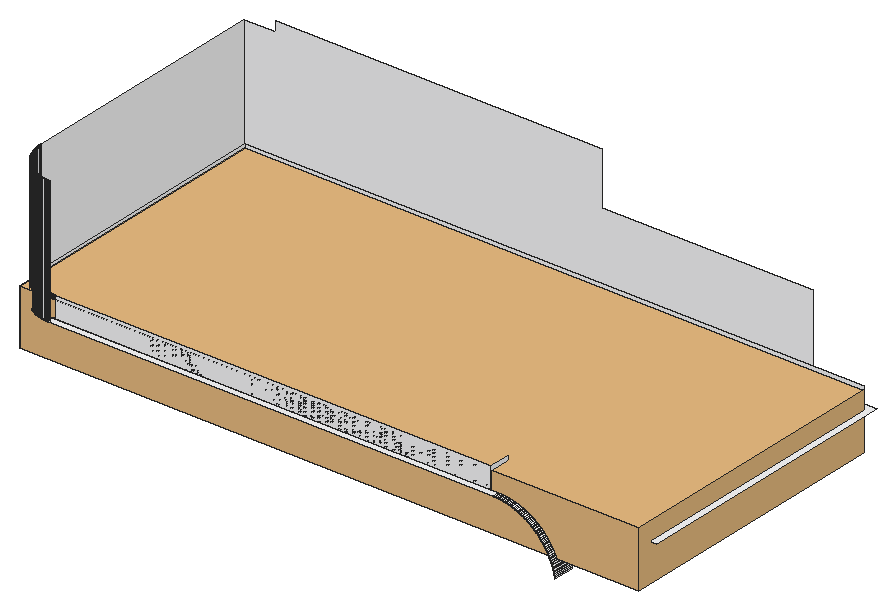
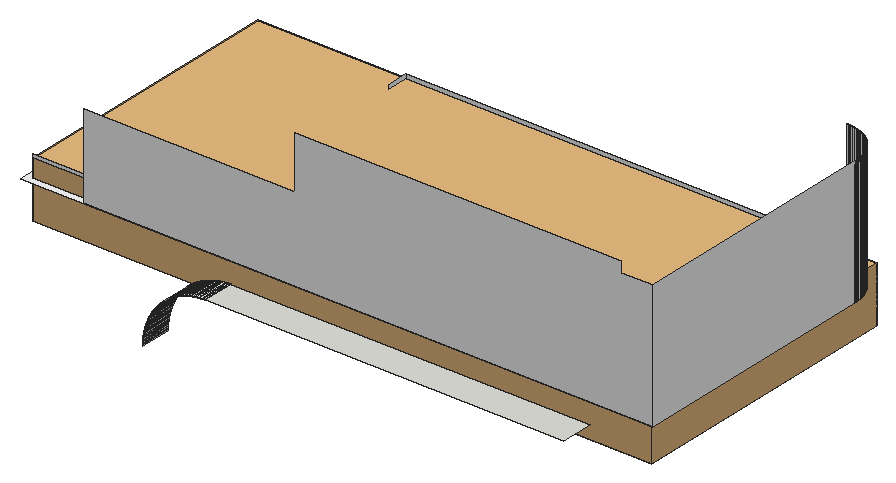
# SketchUp Ruby script. Lengths in inches.
U = 1.inch
M = Sketchup.active_model
def pt(a) = Geom::Point3d.new(a.map { |v| v * U })
def face(e, loops, mat)
  f = e.add_face(loops[0].map { |a| pt(a) })
  loops[1..].each { |l| e.add_face(l.map { |a| pt(a) }).erase! }
  f.material = f.back_material = mat if mat
  f
end
# faces: each face lists its corners as indices into pts; further lists are holes
def faces(e, pts, list, mat = nil) = list.each { |f| face(e, (f[0].is_a?(Array) ? f : [f]).map { |l| l.map { |i| pts[i] } }, mat) }
# xy, xz, yz: faces in a plane at the given z, y or x. An outline is a flat list of corners, or four numbers for a rectangle; further outlines are holes
def ring(l) = l.size == 4 ? [[l[0], l[1]], [l[2], l[1]], [l[2], l[3]], [l[0], l[3]]] : l.each_slice(2).to_a
def flat(e, list, mat, &to3) = list.each { |f| face(e, (f[0].is_a?(Array) ? f : [f]).map { |l| ring(l).map { |u, v| to3.(u, v) } }, mat) }
def xy(e, z, list, mat = nil) = flat(e, list, mat) { |x, y| [x, y, z] }
def xz(e, y, list, mat = nil) = flat(e, list, mat) { |x, z| [x, y, z] }
def yz(e, x, list, mat = nil) = flat(e, list, mat) { |y, z| [x, y, z] }
def lines(e, pts, list) = list.each { |a, b| e.add_line(pt(pts[a]), pt(pts[b])) }
# prism: a flat outline (further loops are holes) pulled along v
def prism(e, loops, v, mat = nil)
  f = face(e, loops, mat); d = Geom::Vector3d.new(v.map { |x| x * U })
  f.pushpull(f.normal.samedirection?(d) ? d.length : -d.length)
end
def box(e, o, s, mat = nil) = prism(e, [[o, [o[0] + s[0], o[1], o[2]], [o[0] + s[0], o[1] + s[1], o[2]], [o[0], o[1] + s[1], o[2]]]], [0, 0, s[2]], mat)
def at(x, y, z, deg = 0) = Geom::Transformation.translation(pt([x, y, z])) * Geom::Transformation.rotation(ORIGIN, Z_AXIS, deg.degrees)
def axes(o, x, y, z) = Geom::Transformation.new([*x, 0, *y, 0, *z, 0, *pt(o).to_a, 1])
def part(name) = M.definitions.add(name)
# library, detail: a bought-in or finely detailed component or shape, given as its bounding box
def library(name, o, s) = part(name).tap { |d| box(d.entities, o, s) }
def detail(e, o, s) = box(e.add_group.entities, o, s)
def put(e, d, t, mat = nil) = e.add_instance(d, t).tap { |i| i.material = mat if mat }
def group(e, t, mat = nil) = e.add_group.tap { |g| g.transformation = t; g.material = mat if mat }.entities
root = M.entities
M.materials.add("[Quartz Light Grey]").color = [251, 251, 252]
c1 = library("Group\#20",[0,0,-16.01],[176,80,16.01])
xy(root,222,[[54,271,156,280],[156,271,156.2,280],[156.2,271,156.4,280]])
xy(root,227.99,[[174.47,187,174.71,193]],"[Quartz Light Grey]")
xy(root,228,[[[47.6875,187,47.53,187.01,47.37,187.02,47.22,187.03,46.9,187.05,46.75,187.07,46.59,187.08,46.43,187.1,46.28,187.125,46.12,187.15,45.97,187.17,45.8125,187.2,45.66,187.23,45.51,187.26,45.35,187.3,45.2,187.33,45.05,187.37,44.89,187.41,44.59,187.49,44.14,187.64,43.99,187.6875,43.85,187.74,43.7,187.8,43.55,187.85,43.41,187.91,43.26,187.97,43.12,188.04,42.98,188.1,42.83,188.17,42.27,188.45,42.14,188.53,42,188.61,41.86,188.6875,41.73,188.77,41.6,188.85,41.46,188.9375,41.33,189.02,41.07,189.2,40.95,189.29,40.82,189.38,40.69,189.48,40.57,189.58,40.45,189.67,40.33,189.77,40.09,189.98,39.97,190.08,39.85,190.1875,39.74,190.3,39.625,190.4,39.51,190.51,39.4,190.625,39.3,190.74,39.1875,190.85,39.08,190.97,38.98,191.09,38.77,191.33,38.67,191.45,38.58,191.57,38.48,191.69,38.38,191.82,38.29,191.95,38.2,192.07,38.02,192.33,37.9375,192.46,37.85,192.6,37.77,192.73,37.6875,192.86,37.61,193,37.53,193.14,37.45,193.27,37.17,193.83,37.1,193.98,37.04,194.12,36.97,194.26,36.91,194.41,36.85,194.55,36.8,194.7,36.74,194.85,36.6875,194.99,36.64,195.14,36.49,195.59,36.41,195.89,36.37,196.05,36.33,196.2,36.3,196.35,36.26,196.51,36.23,196.66,36.2,196.8125,36.17,196.97,36.15,197.12,36.125,197.28,36.1,197.43,36.08,197.59,36.07,197.75,36.05,197.9,36.03,198.22,36.02,198.37,36.01,198.53,36,198.6875,36,271,216,271,216,193,174,193,174,187],[47.74,189,172,189,172,195,214,195,214,269,38,269,38,198.74,38.01,198.61,38.01,198.48,38.03,198.22,38.04,198.08,38.05,197.95,38.09,197.69,38.1,197.57,38.125,197.4375,38.14,197.31,38.17,197.18,38.19,197.05,38.25,196.79,38.28,196.67,38.34,196.41,38.375,196.29,38.41,196.16,38.45,196.03,38.53,195.79,38.57,195.66,38.62,195.54,38.66,195.42,38.71,195.29,38.76,195.17,38.8125,195.05,38.86,194.93,38.92,194.8125,38.97,194.69,39.03,194.58,39.15,194.34,39.21,194.23,39.28,194.11,39.34,194,39.41,193.89,39.47,193.78,39.54,193.66,39.61,193.55,39.69,193.44,39.76,193.34,39.83,193.23,39.91,193.12,39.99,193.02,40.07,192.91,40.23,192.71,40.3125,192.61,40.4,192.51,40.48,192.41,40.66,192.21,40.75,192.12,40.84,192.02,41.02,191.84,41.12,191.75,41.21,191.66,41.41,191.48,41.51,191.4,41.61,191.3125,41.71,191.23,41.91,191.07,42.02,190.99,42.12,190.91,42.23,190.83,42.34,190.76,42.44,190.69,42.55,190.61,42.66,190.54,42.78,190.47,42.89,190.41,43,190.34,43.11,190.28,43.23,190.21,43.34,190.15,43.58,190.03,43.69,189.97,43.8125,189.92,43.93,189.86,44.05,189.8125,44.17,189.76,44.29,189.71,44.42,189.66,44.54,189.62,44.66,189.57,44.79,189.53,45.03,189.45,45.16,189.41,45.29,189.375,45.41,189.34,45.67,189.28,45.79,189.25,46.05,189.19,46.18,189.17,46.31,189.14,46.4375,189.125,46.57,189.1,46.69,189.09,46.95,189.05,47.08,189.04,47.22,189.03,47.48,189.01,47.61,189.01]],[174,187,174.24,193]],"[Quartz Light Grey]")
xz(root,187,[[47.6875,228,47.84,264],[47.84,228,48,264]],"[Quartz Light Grey]")
xz(root,189,[[47.74,228,47.87,234],[47.87,228,48,234],[48,228,172,234]],"[Quartz Light Grey]")
xz(root,189.01,[[47.48,228,47.61,234]],"[Quartz Light Grey]")
xz(root,269,[[38,228,214,234]],"[Quartz Light Grey]")
xz(root,271,[[36,228,36,264,45,264,45,267,138,267,138,252,198,252,198,228]],"[Quartz Light Grey]")
yz(root,36,[[198.6875,228,198.84,264],[198.84,228,199,264],[199,228,271,264]],"[Quartz Light Grey]")
yz(root,38,[[198.74,228,198.87,234],[198.87,228,199,234],[199,228,269,234]],"[Quartz Light Grey]")
yz(root,38.01,[[198.48,228,198.61,234]],"[Quartz Light Grey]")
yz(root,172,[[189,228,195,234]],"[Quartz Light Grey]")
yz(root,174,[[271,204,280,204.2],[271,204.2,280,204.4]])
p = [[174,271,204.4],[173.99,271,204.61],[173.99,280,204.61],[174,280,204.4],[173.98,271,204.81],[173.98,280,204.81],
  [173.97,271,205.01],[173.97,280,205.01],[173.96,271,205.21],[173.96,280,205.21],[173.94,271,205.41],[173.94,280,205.41],
  [173.93,271,205.61],[173.93,280,205.61],[173.91,271,205.81],[173.91,280,205.81],[173.89,271,206.02],[173.89,280,206.02],
  [173.86,271,206.22],[173.86,280,206.22],[173.84,271,206.42],[173.84,280,206.42],[173.81,271,206.62],[173.81,280,206.62],
  [173.78,271,206.82],[173.78,280,206.82],[173.75,271,207.02],[173.75,280,207.02],[173.71,271,207.21],[173.71,280,207.21],
  [173.67,271,207.41],[173.67,280,207.41],[173.63,271,207.61],[173.63,280,207.61],[173.59,271,207.81],[173.59,280,207.81],
  [173.55,271,208.01],[173.55,280,208.01],[173.5,271,208.2],[173.5,280,208.2],[173.45,271,208.4],[173.45,280,208.4],
  [173.4,271,208.59],[173.4,280,208.59],[173.35,271,208.79],[173.35,280,208.79],[173.3,271,208.98],[173.3,280,208.98],
  [173.24,271,209.18],[173.24,280,209.18],[173.18,271,209.37],[173.18,280,209.37],[173.12,271,209.5625],[173.12,280,209.5625],
  [173.06,271,209.75],[173.06,280,209.75],[172.99,271,209.95],[172.99,280,209.95],[172.92,271,210.14],[172.92,280,210.14],
  [172.85,271,210.32],[172.85,280,210.32],[172.78,271,210.51],[172.78,280,210.51],[172.71,271,210.7],[172.71,280,210.7],
  [172.63,271,210.89],[172.63,280,210.89],[172.55,271,211.07],[172.55,280,211.07],[172.47,271,211.26],[172.47,280,211.26],
  [172.39,271,211.44],[172.39,280,211.44],[172.3,271,211.63],[172.3,280,211.63],[172.22,271,211.81],[172.22,280,211.81],
  [172.13,271,211.99],[172.13,280,211.99],[172.04,271,212.17],[172.04,280,212.17],[171.95,271,212.35],[171.95,280,212.35],
  [171.85,271,212.53],[171.85,280,212.53],[171.75,271,212.71],[171.75,280,212.71],[171.66,271,212.88],[171.66,280,212.88],
  [171.55,271,213.06],[171.55,280,213.06],[191.7,187,213.28],[191.7,193,213.28],[191.74,193,213.05],[191.74,187,213.05],
  [171.45,271,213.23],[171.45,280,213.23],[171.35,271,213.4],[171.35,280,213.4],[191.65,187,213.51],[191.65,193,213.51],
  [171.24,271,213.58],[171.24,280,213.58],[191.61,187,213.74],[191.61,193,213.74],[171.13,271,213.75],[171.13,280,213.75],
  [191.56,187,213.97],[191.56,193,213.97],[171.02,271,213.92],[171.02,280,213.92],[170.91,271,214.08],[170.91,280,214.08],
  [191.5,187,214.2],[191.5,193,214.2],[170.8,271,214.25],[170.8,280,214.25],[191.45,187,214.43],[191.45,193,214.43],
  [170.68,271,214.42],[170.68,280,214.42],[191.39,187,214.66],[191.39,193,214.66],[170.5625,271,214.58],[170.5625,280,214.58],
  [170.44,271,214.74],[170.44,280,214.74],[191.32,187,214.89],[191.32,193,214.89],[170.32,271,214.9],[170.32,280,214.9],
  [191.26,187,215.11],[191.26,193,215.11],[170.2,271,215.0625],[170.2,280,215.0625],[191.19,187,215.34],[191.19,193,215.34],
  [170.07,271,215.22],[170.07,280,215.22],[169.95,271,215.38],[169.95,280,215.38],[191.12,187,215.5625],[191.12,193,215.5625],
  [169.82,271,215.54],[169.82,280,215.54],[169.6875,271,215.69],[169.6875,280,215.69],[191.04,187,215.79],[191.04,193,215.79],
  [169.56,271,215.84],[169.56,280,215.84],[190.97,187,216.01],[190.97,193,216.01],[169.42,271,215.99],[169.42,280,215.99],
  [190.89,187,216.23],[190.89,193,216.23],[169.29,271,216.14],[169.29,280,216.14],[169.15,271,216.29],[169.15,280,216.29],
  [190.8,187,216.45],[190.8,193,216.45],[169.01,271,216.4375],[169.01,280,216.4375],[168.87,271,216.58],[168.87,280,216.58],
  [190.72,187,216.67],[190.72,193,216.67],[168.73,271,216.73],[168.73,280,216.73],[190.63,187,216.89],[190.63,193,216.89],
  [168.58,271,216.87],[168.58,280,216.87],[190.54,187,217.11],[190.54,193,217.11],[168.4375,271,217.01],[168.4375,280,217.01],
  [168.29,271,217.15],[168.29,280,217.15],[190.44,187,217.32],[190.44,193,217.32],[168.14,271,217.29],[168.14,280,217.29],
  [190.35,187,217.54],[190.35,193,217.54],[167.99,271,217.42],[167.99,280,217.42],[167.84,271,217.56],[167.84,280,217.56],
  [190.25,187,217.75],[190.25,193,217.75],[167.69,271,217.6875],[167.69,280,217.6875],[190.14,187,217.96],[190.14,193,217.96],
  [167.54,271,217.82],[167.54,280,217.82],[167.38,271,217.95],[167.38,280,217.95],[167.22,271,218.07],[167.22,280,218.07],
  [190.04,187,218.17],[190.04,193,218.17],[167.0625,271,218.2],[167.0625,280,218.2],[189.93,187,218.38],[189.93,193,218.38],
  [166.9,271,218.32],[166.9,280,218.32],[166.74,271,218.44],[166.74,280,218.44],[189.82,187,218.59],[189.82,193,218.59],
  [166.58,271,218.5625],[166.58,280,218.5625],[189.7,187,218.8],[189.7,193,218.8],[166.42,271,218.68],[166.42,280,218.68],
  [166.25,271,218.8],[166.25,280,218.8],[189.59,187,219],[189.59,193,219],[166.08,271,218.91],[166.08,280,218.91],
  [165.92,271,219.02],[165.92,280,219.02],[189.47,187,219.2],[189.47,193,219.2],[165.75,271,219.13],[165.75,280,219.13],
  [165.58,271,219.24],[165.58,280,219.24],[189.35,187,219.4],[189.35,193,219.4],[165.4,271,219.35],[165.4,280,219.35],
  [165.23,271,219.45],[165.23,280,219.45],[189.22,187,219.61],[189.22,193,219.61],[165.06,271,219.55],[165.06,280,219.55],
  [189.1,187,219.8],[189.1,193,219.8],[164.88,271,219.66],[164.88,280,219.66],[164.71,271,219.75],[164.71,280,219.75],
  [188.97,187,220],[188.97,193,220],[164.53,271,219.85],[164.53,280,219.85],[164.35,271,219.95],[164.17,271,220.04],
  [164.17,280,220.04],[164.35,280,219.95],[188.83,187,220.2],[188.83,193,220.2],[163.99,271,220.13],[163.99,280,220.13],
  [163.81,271,220.22],[163.81,280,220.22],[188.7,187,220.39],[188.7,193,220.39],[163.63,271,220.3],[163.63,280,220.3],
  [163.44,271,220.39],[163.44,280,220.39],[188.5625,187,220.58],[188.5625,193,220.58],[163.26,271,220.47],[163.26,280,220.47],
  [163.07,271,220.55],[163.07,280,220.55],[188.42,187,220.77],[188.42,193,220.77],[162.89,271,220.63],[162.7,271,220.71],
  [162.7,280,220.71],[162.89,280,220.63],[162.51,271,220.78],[162.51,280,220.78],[188.28,187,220.96],[188.28,193,220.96],
  [162.32,271,220.85],[162.32,280,220.85],[162.14,271,220.92],[161.95,271,220.99],[161.95,280,220.99],[162.14,280,220.92],
  [188.14,187,221.14],[188.14,193,221.14],[161.75,271,221.06],[161.75,280,221.06],[187.99,187,221.33],[187.99,193,221.33],
  [161.5625,271,221.12],[161.37,271,221.18],[161.37,280,221.18],[161.5625,280,221.12],[161.18,271,221.24],[160.98,271,221.3],
  [160.98,280,221.3],[161.18,280,221.24],[187.84,187,221.51],[187.84,193,221.51],[160.79,271,221.35],[160.79,280,221.35],
  [160.59,271,221.4],[160.4,271,221.45],[160.4,280,221.45],[160.59,280,221.4],[187.6875,187,221.69],[187.6875,193,221.69],
  [160.01,271,221.55],[159.81,271,221.59],[159.81,280,221.59],[160.01,280,221.55],[160.2,271,221.5],[160.2,280,221.5],
  [159.61,271,221.63],[159.41,271,221.67],[159.41,280,221.67],[159.61,280,221.63],[187.53,187,221.87],[187.53,193,221.87],
  [159.02,271,221.75],[158.82,271,221.78],[158.82,280,221.78],[159.02,280,221.75],[159.21,271,221.71],[159.21,280,221.71],
  [158.42,271,221.84],[158.22,271,221.86],[158.22,280,221.86],[158.42,280,221.84],[158.62,271,221.81],[158.62,280,221.81],
  [187.375,187,222.04],[187.375,193,222.04],[157.41,271,221.94],[157.21,271,221.96],[157.21,280,221.96],[157.41,280,221.94],
  [157.61,271,221.93],[157.61,280,221.93],[157.81,271,221.91],[157.81,280,221.91],[158.02,271,221.89],[158.02,280,221.89],
  [187.22,187,222.22],[187.22,193,222.22],[156.61,271,221.99],[156.4,271,222],[156.4,280,222],[156.61,280,221.99],
  [156.81,271,221.98],[156.81,280,221.98],[157.01,271,221.97],[157.01,280,221.97],[187.06,187,222.39],[187.06,193,222.39],
  [186.89,187,222.56],[186.89,193,222.56],[186.73,187,222.73],[186.73,193,222.73],[186.56,187,222.89],[186.56,193,222.89],
  [186.39,187,223.06],[186.39,193,223.06],[186.22,187,223.22],[186.22,193,223.22],[186.04,187,223.375],[186.04,193,223.375],
  [185.87,187,223.53],[185.87,193,223.53],[185.69,187,223.6875],[185.69,193,223.6875],[185.51,187,223.84],[185.51,193,223.84],
  [185.33,187,223.99],[185.33,193,223.99],[185.14,187,224.14],[185.14,193,224.14],[184.96,187,224.28],[184.96,193,224.28],
  [184.77,187,224.42],[184.77,193,224.42],[184.58,187,224.5625],[184.58,193,224.5625],[184.39,187,224.7],[184.39,193,224.7],
  [184.2,187,224.83],[184.2,193,224.83],[184,187,224.97],[184,193,224.97],[183.8,187,225.1],[183.8,193,225.1],
  [183.61,187,225.22],[183.61,193,225.22],[183.4,187,225.35],[183.4,193,225.35],[183.2,187,225.47],[183.2,193,225.47],
  [183,187,225.59],[183,193,225.59],[182.8,187,225.7],[182.8,193,225.7],[182.59,187,225.82],[182.59,193,225.82],
  [182.38,187,225.93],[182.38,193,225.93],[182.17,187,226.04],[182.17,193,226.04],[181.96,187,226.14],[181.96,193,226.14],
  [181.75,187,226.25],[181.75,193,226.25],[181.54,187,226.35],[181.54,193,226.35],[181.32,187,226.44],[181.32,193,226.44],
  [181.11,187,226.54],[181.11,193,226.54],[180.89,187,226.63],[180.89,193,226.63],[180.67,187,226.72],[180.67,193,226.72],
  [180.45,187,226.8],[180.45,193,226.8],[180.23,187,226.89],[180.23,193,226.89],[180.01,187,226.97],[180.01,193,226.97],
  [179.5625,187,227.12],[179.5625,193,227.12],[179.79,193,227.04],[179.79,187,227.04],[179.34,187,227.19],[179.34,193,227.19],
  [179.11,187,227.26],[179.11,193,227.26],[178.66,187,227.39],[178.66,193,227.39],[178.89,193,227.32],[178.89,187,227.32],
  [178.2,187,227.5],[178.2,193,227.5],[178.43,193,227.45],[178.43,187,227.45],[177.97,187,227.56],[177.97,193,227.56],
  [177.51,187,227.65],[177.51,193,227.65],[177.74,193,227.61],[177.74,187,227.61],[176.82,187,227.78],[176.82,193,227.78],
  [177.05,193,227.74],[177.05,187,227.74],[177.28,193,227.7],[177.28,187,227.7],[176.12,187,227.875],[176.12,193,227.875],
  [176.35,193,227.85],[176.35,187,227.85],[176.58,193,227.8125],[176.58,187,227.8125],[175.18,187,227.96],[175.18,193,227.96],
  [175.41,193,227.94],[175.41,187,227.94],[175.65,193,227.92],[175.65,187,227.92],[175.88,193,227.9],[175.88,187,227.9],
  [47.06,187.04,264],[46.9,187.05,264],[46.9,187.05,228],[47.06,187.04,228],[47.22,187.03,264],[47.22,187.03,228],
  [47.37,187.02,264],[47.37,187.02,228],[47.53,187.01,264],[47.53,187.01,228],[47.6875,187,264],[47.6875,187,228],
  [174.24,187,228],[174.24,193,228],[174.47,193,227.99],[174.47,187,227.99],[174.71,187,227.99],[174.71,193,227.99],
  [174.94,193,227.98],[174.94,187,227.98],[46.12,187.15,264],[45.97,187.17,264],[45.97,187.17,228],[46.12,187.15,228],
  [46.28,187.125,264],[46.28,187.125,228],[46.43,187.1,264],[46.43,187.1,228],[46.59,187.08,264],[46.59,187.08,228],
  [46.75,187.07,264],[46.75,187.07,228],[45.66,187.23,264],[45.51,187.26,264],[45.51,187.26,228],[45.66,187.23,228],
  [45.8125,187.2,264],[45.8125,187.2,228],[45.2,187.33,264],[45.05,187.37,264],[45.05,187.37,228],[45.2,187.33,228],
  [45.35,187.3,264],[45.35,187.3,228],[44.89,187.41,264],[44.74,187.45,264],[44.74,187.45,228],[44.89,187.41,228],
  [44.44,187.54,264],[44.29,187.59,264],[44.29,187.59,228],[44.44,187.54,228],[44.59,187.49,264],[44.59,187.49,228],
  [44.14,187.64,264],[43.99,187.6875,264],[43.99,187.6875,228],[44.14,187.64,228],[43.85,187.74,264],[43.7,187.8,264],
  [43.7,187.8,228],[43.85,187.74,228],[43.55,187.85,264],[43.55,187.85,228],[43.41,187.91,264],[43.26,187.97,264],
  [43.26,187.97,228],[43.41,187.91,228],[43.12,188.04,264],[42.98,188.1,264],[42.98,188.1,228],[43.12,188.04,228],
  [42.83,188.17,264],[42.83,188.17,228],[42.69,188.24,264],[42.55,188.31,264],[42.55,188.31,228],[42.69,188.24,228],
  [42.41,188.38,264],[42.41,188.38,228],[42.27,188.45,264],[42.27,188.45,228],[42.14,188.53,264],[42,188.61,264],
  [42,188.61,228],[42.14,188.53,228],[41.86,188.6875,264],[41.86,188.6875,228],[41.73,188.77,264],[41.73,188.77,228],
  [41.6,188.85,264],[41.6,188.85,228],[41.46,188.9375,264],[41.33,189.02,264],[41.33,189.02,228],[41.46,188.9375,228],
  [41.2,189.11,264],[41.2,189.11,228],[47.08,189.04,228],[46.95,189.05,228],[46.95,189.05,234],[47.08,189.04,234],
  [47.22,189.03,228],[47.22,189.03,234],[47.35,189.02,228],[47.35,189.02,234],[47.48,189.01,228],[47.48,189.01,234],
  [47.74,189,228],[47.61,189.01,228],[47.61,189.01,234],[47.74,189,234],[41.07,189.2,264],[41.07,189.2,228],
  [46.31,189.14,228],[46.18,189.17,228],[46.18,189.17,234],[46.31,189.14,234],[46.4375,189.125,228],[46.4375,189.125,234],
  [46.57,189.1,228],[46.57,189.1,234],[46.69,189.09,228],[46.69,189.09,234],[46.82,189.07,228],[46.82,189.07,234],
  [40.95,189.29,264],[40.95,189.29,228],[45.79,189.25,228],[45.67,189.28,228],[45.67,189.28,234],[45.79,189.25,234],
  [45.92,189.22,228],[45.92,189.22,234],[46.05,189.19,228],[46.05,189.19,234],[40.82,189.38,264],[40.82,189.38,228],
  [45.41,189.34,228],[45.29,189.375,228],[45.29,189.375,234],[45.41,189.34,234],[45.54,189.31,228],[45.54,189.31,234],
  [40.69,189.48,264],[40.69,189.48,228],[45.03,189.45,228],[44.91,189.49,228],[44.91,189.49,234],[45.03,189.45,234],
  [45.16,189.41,228],[45.16,189.41,234],[40.57,189.58,264],[40.57,189.58,228],[44.79,189.53,228],[44.66,189.57,228],
  [44.66,189.57,234],[44.79,189.53,234],[40.45,189.67,264],[40.45,189.67,228],[44.54,189.62,228],[44.42,189.66,228],
  [44.42,189.66,234],[44.54,189.62,234],[40.33,189.77,264],[40.33,189.77,228],[44.29,189.71,228],[44.17,189.76,228],
  [44.17,189.76,234],[44.29,189.71,234],[40.21,189.875,264],[40.21,189.875,228],[44.05,189.8125,228],[43.93,189.86,228],
  [43.93,189.86,234],[44.05,189.8125,234],[40.09,189.98,264],[40.09,189.98,228],[43.8125,189.92,228],[43.69,189.97,228],
  [43.69,189.97,234],[43.8125,189.92,234],[39.97,190.08,264],[39.97,190.08,228],[43.58,190.03,228],[43.46,190.09,228],
  [43.46,190.09,234],[43.58,190.03,234],[39.85,190.1875,264],[39.85,190.1875,228],[43.34,190.15,228],[43.34,190.15,234],
  [39.74,190.3,264],[39.74,190.3,228],[43.23,190.21,228],[43.11,190.28,228],[43.11,190.28,234],[43.23,190.21,234],
  [39.625,190.4,264],[39.625,190.4,228],[43,190.34,228],[42.89,190.41,228],[42.89,190.41,234],[43,190.34,234],
  [39.51,190.51,264],[39.51,190.51,228],[42.78,190.47,228],[42.78,190.47,234],[39.4,190.625,264],[39.4,190.625,228],
  [42.66,190.54,228],[42.55,190.61,228],[42.55,190.61,234],[42.66,190.54,234],[39.3,190.74,264],[39.3,190.74,228],
  [42.44,190.69,228],[42.44,190.69,234],[39.1875,190.85,264],[39.1875,190.85,228],[42.34,190.76,228],[42.34,190.76,234],
  [42.23,190.83,228],[42.12,190.91,228],[42.12,190.91,234],[42.23,190.83,234],[39.08,190.97,264],[39.08,190.97,228],
  [42.02,190.99,228],[42.02,190.99,234],[38.98,191.09,264],[38.98,191.09,228],[41.91,191.07,228],[41.91,191.07,234],
  [38.875,191.21,264],[38.875,191.21,228],[41.81,191.15,228],[41.71,191.23,228],[41.71,191.23,234],[41.81,191.15,234],
  [38.77,191.33,264],[38.77,191.33,228],[41.61,191.3125,228],[41.61,191.3125,234],[38.67,191.45,264],[38.67,191.45,228],
  [41.51,191.4,228],[41.51,191.4,234],[38.58,191.57,264],[38.58,191.57,228],[41.41,191.48,228],[41.41,191.48,234],
  [41.31,191.57,228],[41.31,191.57,234],[38.48,191.69,264],[38.48,191.69,228],[41.21,191.66,228],[41.21,191.66,234],
  [38.38,191.82,264],[38.38,191.82,228],[41.12,191.75,228],[41.02,191.84,228],[41.02,191.84,234],[41.12,191.75,234],
  [38.29,191.95,264],[38.29,191.95,228],[40.93,191.93,228],[40.93,191.93,234],[38.2,192.07,264],[38.2,192.07,228],
  [40.84,192.02,228],[40.84,192.02,234],[40.75,192.12,228],[40.75,192.12,234],[38.11,192.2,264],[38.11,192.2,228],
  [40.66,192.21,228],[40.66,192.21,234],[38.02,192.33,264],[38.02,192.33,228],[40.57,192.31,228],[40.57,192.31,234],
  [37.9375,192.46,264],[37.9375,192.46,228],[40.48,192.41,228],[40.48,192.41,234],[40.4,192.51,228],[40.4,192.51,234],
  [37.85,192.6,264],[37.85,192.6,228],[40.3125,192.61,228],[40.3125,192.61,234],[37.77,192.73,264],[37.77,192.73,228],
  [40.23,192.71,228],[40.23,192.71,234],[37.6875,192.86,264],[37.6875,192.86,228],[40.15,192.81,228],[40.15,192.81,234],
  [40.07,192.91,228],[40.07,192.91,234],[37.61,193,264],[37.61,193,228],[39.99,193.02,228],[39.99,193.02,234],
  [37.53,193.14,264],[37.53,193.14,228],[39.91,193.12,228],[39.91,193.12,234],[37.45,193.27,264],[37.45,193.27,228],
  [39.83,193.23,228],[39.83,193.23,234],[39.76,193.34,228],[39.76,193.34,234],[37.38,193.41,264],[37.38,193.41,228],
  [39.69,193.44,228],[39.69,193.44,234],[37.31,193.55,264],[37.31,193.55,228],[39.61,193.55,228],[39.61,193.55,234],
  [37.24,193.69,264],[37.24,193.69,228],[39.54,193.66,228],[39.54,193.66,234],[37.17,193.83,264],[37.17,193.83,228],
  [39.47,193.78,228],[39.47,193.78,234],[37.1,193.98,264],[37.1,193.98,228],[39.41,193.89,228],[39.41,193.89,234],
  [39.34,194,228],[39.34,194,234],[37.04,194.12,264],[37.04,194.12,228],[39.28,194.11,228],[39.28,194.11,234],
  [36.97,194.26,264],[36.97,194.26,228],[39.21,194.23,228],[39.21,194.23,234],[39.15,194.34,228],[39.15,194.34,234],
  [36.91,194.41,264],[36.91,194.41,228],[39.09,194.46,228],[39.09,194.46,234],[36.85,194.55,264],[36.85,194.55,228],
  [39.03,194.58,228],[39.03,194.58,234],[36.8,194.7,264],[36.8,194.7,228],[38.97,194.69,228],[38.97,194.69,234],
  [36.74,194.85,264],[36.74,194.85,228],[38.92,194.8125,228],[38.92,194.8125,234],[36.6875,194.99,264],[36.6875,194.99,228],
  [38.86,194.93,228],[38.86,194.93,234],[38.8125,195.05,228],[38.8125,195.05,234],[36.64,195.14,264],[36.64,195.14,228],
  [36.59,195.29,264],[36.59,195.29,228],[38.76,195.17,228],[38.76,195.17,234],[38.71,195.29,228],[38.71,195.29,234],
  [36.54,195.44,264],[36.54,195.44,228],[38.66,195.42,228],[38.66,195.42,234],[36.49,195.59,264],[36.49,195.59,228],
  [38.62,195.54,228],[38.62,195.54,234],[38.57,195.66,228],[38.57,195.66,234],[36.45,195.74,264],[36.45,195.74,228],
  [36.41,195.89,264],[36.41,195.89,228],[38.53,195.79,228],[38.53,195.79,234],[38.49,195.91,228],[38.49,195.91,234],
  [36.37,196.05,264],[36.37,196.05,228],[38.45,196.03,228],[38.45,196.03,234],[36.33,196.2,264],[36.33,196.2,228],
  [38.41,196.16,228],[38.41,196.16,234],[36.3,196.35,264],[36.3,196.35,228],[38.375,196.29,228],[38.375,196.29,234],
  [38.34,196.41,228],[38.34,196.41,234],[36.26,196.51,264],[36.26,196.51,228],[38.31,196.54,228],[38.31,196.54,234],
  [36.23,196.66,264],[36.23,196.66,228],[38.28,196.67,228],[38.28,196.67,234],[36.2,196.8125,264],[36.2,196.8125,228],
  [38.25,196.79,228],[38.25,196.79,234],[36.17,196.97,264],[36.17,196.97,228],[38.22,196.92,228],[38.22,196.92,234],
  [38.19,197.05,228],[38.19,197.05,234],[36.15,197.12,264],[36.15,197.12,228],[38.17,197.18,228],[38.17,197.18,234],
  [36.125,197.28,264],[36.125,197.28,228],[38.14,197.31,228],[38.14,197.31,234],[36.1,197.43,264],[36.1,197.43,228],
  [38.125,197.4375,228],[38.125,197.4375,234],[36.08,197.59,264],[36.08,197.59,228],[38.1,197.57,228],[38.1,197.57,234],
  [36.07,197.75,264],[36.07,197.75,228],[38.09,197.69,228],[38.09,197.69,234],[36.05,197.9,264],[36.05,197.9,228],
  [38.07,197.82,228],[38.07,197.82,234],[38.05,197.95,228],[38.05,197.95,234],[36.04,198.06,264],[36.04,198.06,228],
  [38.04,198.08,228],[38.04,198.08,234],[36.03,198.22,264],[36.03,198.22,228],[38.03,198.22,228],[38.03,198.22,234],
  [36.02,198.37,264],[36.02,198.37,228],[38.02,198.35,228],[38.02,198.35,234],[38.01,198.48,228],[38.01,198.48,234],
  [36.01,198.53,264],[36.01,198.53,228],[36,198.6875,264],[36,198.6875,228],[38.01,198.61,228],[38,198.74,228],
  [38,198.74,234],[38.01,198.61,234]]
faces(root,p,[[0,1,2,3],[1,4,5,2],[4,6,7,5],[6,8,9,7],[8,10,11,9],[10,12,13,11],[12,14,15,13],[14,16,17,15],
  [16,18,19,17],[18,20,21,19],[20,22,23,21],[22,24,25,23],[24,26,27,25],[26,28,29,27],[28,30,31,29],[30,32,33,31],
  [32,34,35,33],[34,36,37,35],[36,38,39,37],[38,40,41,39],[40,42,43,41],[42,44,45,43],[44,46,47,45],[46,48,49,47],
  [48,50,51,49],[50,52,53,51],[52,54,55,53],[54,56,57,55],[56,58,59,57],[58,60,61,59],[60,62,63,61],[62,64,65,63],
  [64,66,67,65],[66,68,69,67],[68,70,71,69],[70,72,73,71],[72,74,75,73],[74,76,77,75],[76,78,79,77],[78,80,81,79],
  [80,82,83,81],[82,84,85,83],[84,86,87,85],[86,88,89,87],[88,90,91,89],[90,96,97,91],[96,98,99,97],[98,102,103,99],
  [102,106,107,103],[106,110,111,107],[110,112,113,111],[112,116,117,113],[116,120,121,117],[120,124,125,121],[124,126,127,125],[126,130,131,127],
  [130,134,135,131],[134,138,139,135],[138,140,141,139],[140,144,145,141],[144,146,147,145],[146,150,151,147],[150,154,155,151],[154,158,159,155],
  [158,160,161,159],[160,164,165,161],[164,166,167,165],[166,170,171,167],[170,174,175,171],[174,178,179,175],[178,180,181,179],[180,184,185,181],
  [184,188,189,185],[188,190,191,189],[190,194,195,191],[194,198,199,195],[198,200,201,199],[200,202,203,201],[202,206,207,203],[206,210,211,207],
  [210,212,213,211],[212,216,217,213],[216,220,221,217],[220,222,223,221],[222,226,227,223],[226,228,229,227],[228,232,233,229],[232,234,235,233],
  [234,238,239,235],[238,240,241,239],[240,244,245,241],[244,248,249,245],[248,250,251,249],[250,254,255,251],[256,257,258,259],[254,256,259,255],
  [257,262,263,258],[262,264,265,263],[264,268,269,265],[268,270,271,269],[270,274,275,271],[274,276,277,275],[280,281,282,283],[276,280,283,277],
  [281,284,285,282],[284,288,289,285],[290,291,292,293],[288,290,293,289],[291,296,297,292],[300,301,302,303],[296,300,303,297],[304,305,306,307],
  [301,304,307,302],[305,310,311,306],[312,313,314,315],[310,312,315,311],[318,319,320,321],[322,318,321,323],[313,322,323,314],[324,325,326,327],
  [319,324,327,320],[330,331,332,333],[334,330,333,335],[325,334,335,326],[336,337,338,339],[340,336,339,341],[331,340,341,332],[344,345,346,347],
  [348,344,347,349],[350,348,349,351],[352,350,351,353],[337,352,353,338],[356,357,358,359],[360,356,359,361],[362,360,361,363],[345,362,363,346]])
faces(root,p,[[92,93,94,95],[100,101,93,92],[104,105,101,100],[108,109,105,104],[114,115,109,108],[118,119,115,114],[122,123,119,118],[128,129,123,122],
  [132,133,129,128],[136,137,133,132],[142,143,137,136],[148,149,143,142],[152,153,149,148],[156,157,153,152],[162,163,157,156],[168,169,163,162],
  [172,173,169,168],[176,177,173,172],[182,183,177,176],[186,187,183,182],[192,193,187,186],[196,197,193,192],[204,205,197,196],[208,209,205,204],
  [214,215,209,208],[218,219,215,214],[224,225,219,218],[230,231,225,224],[236,237,231,230],[242,243,237,236],[246,247,243,242],[252,253,247,246],
  [260,261,253,252],[266,267,261,260],[272,273,267,266],[278,279,273,272],[286,287,279,278],[294,295,287,286],[298,299,295,294],[308,309,299,298],
  [316,317,309,308],[328,329,317,316],[342,343,329,328],[354,355,343,342],[364,365,355,354],[366,367,365,364],[368,369,367,366],[370,371,369,368],
  [372,373,371,370],[374,375,373,372],[376,377,375,374],[378,379,377,376],[380,381,379,378],[382,383,381,380],[384,385,383,382],[386,387,385,384],
  [388,389,387,386],[390,391,389,388],[392,393,391,390],[394,395,393,392],[396,397,395,394],[398,399,397,396],[400,401,399,398],[402,403,401,400],
  [404,405,403,402],[406,407,405,404],[408,409,407,406],[410,411,409,408],[412,413,411,410],[414,415,413,412],[416,417,415,414],[418,419,417,416],
  [420,421,419,418],[422,423,421,420],[424,425,423,422],[426,427,425,424],[428,429,427,426],[430,431,429,428],[432,433,431,430],[434,435,433,432],
  [436,437,435,434],[438,439,440,441],[441,440,437,436],[442,443,439,438],[444,445,443,442],[446,447,448,449],[449,448,445,444],[450,451,452,453],
  [453,452,447,446],[454,455,451,450],[456,457,458,459],[459,458,455,454],[460,461,462,463],[463,462,464,465],[465,464,457,456],[466,467,468,469],
  [469,468,470,471],[471,470,461,460],[472,473,474,475],[475,474,476,477],[477,476,478,479],[479,478,467,466],[480,481,482,483],[484,480,483,485],
  [486,484,485,487],[488,486,487,489],[490,488,489,491],[492,493,494,495],[496,497,498,499],[499,498,473,472],[500,501,502,503],[504,500,503,505],
  [506,504,505,507],[508,506,507,509],[510,508,509,511],[481,510,511,482],[512,513,514,515],[516,512,515,517],[501,516,517,502],[518,519,520,521],
  [522,518,521,523],[513,522,523,514],[524,525,526,527],[519,524,527,520],[528,529,530,531],[532,528,531,533],[525,532,533,526],[534,535,536,537],
  [529,534,537,530],[538,539,540,541],[535,538,541,536],[539,542,543,540],[544,545,546,547],[542,544,547,543],[548,549,550,551],[545,548,551,546],
  [549,552,553,550],[554,555,556,557],[552,554,557,553],[555,558,559,556],[558,560,561,559],[562,563,564,565],[560,562,565,561],[563,566,567,564],
  [566,568,569,567],[568,570,571,569],[572,573,574,575],[570,572,575,571],[573,576,577,574],[578,579,580,581],[582,578,581,583],[584,582,583,585],
  [586,584,585,587],[588,589,590,591],[576,592,593,577],[594,595,596,597],[598,594,597,599],[600,598,599,601],[602,600,601,603],[604,602,603,605],
  [579,604,605,580],[592,606,607,593],[608,609,610,611],[612,608,611,613],[614,612,613,615],[595,614,615,596],[606,616,617,607],[618,619,620,621],
  [622,618,621,623],[609,622,623,610],[616,624,625,617],[626,627,628,629],[630,626,629,631],[619,630,631,620],[624,632,633,625],[634,635,636,637],
  [627,634,637,628],[632,638,639,633],[640,641,642,643],[635,640,643,636],[638,644,645,639],[646,647,648,649],[641,646,649,642],[644,650,651,645],
  [652,653,654,655],[647,652,655,648],[650,656,657,651],[658,659,660,661],[653,658,661,654],[656,662,663,657],[664,665,666,667],[659,664,667,660],
  [662,668,669,663],[665,670,671,666],[668,672,673,669],[674,675,676,677],[670,674,677,671],[672,678,679,673],[680,681,682,683],[675,680,683,676],
  [678,684,685,679],[681,686,687,682],[684,688,689,685],[690,691,692,693],[686,690,693,687],[688,694,695,689],[691,696,697,692],[694,698,699,695],
  [696,700,701,697],[702,703,704,705],[700,702,705,701],[698,706,707,699],[703,708,709,704],[706,710,711,707],[708,712,713,709],[710,714,715,711],
  [716,717,718,719],[712,716,719,713],[714,720,721,715],[717,722,723,718],[720,724,725,721],[722,726,727,723],[724,728,729,725],[726,730,731,727],
  [730,732,733,731],[728,734,735,729],[732,736,737,733],[734,738,739,735],[740,741,742,743],[736,740,743,737],[738,744,745,739],[741,746,747,742],
  [744,748,749,745],[746,750,751,747],[750,752,753,751],[748,754,755,749],[752,756,757,753],[754,758,759,755],[756,760,761,757],[758,762,763,759],
  [760,764,765,761],[764,766,767,765],[762,768,769,763],[766,770,771,767],[768,772,773,769],[770,774,775,771],[772,776,777,773],[774,778,779,775],
  [778,780,781,779],[776,782,783,777],[780,784,785,781],[782,786,787,783],[784,788,789,785],[786,790,791,787],[788,792,793,789],[792,794,795,793],
  [790,796,797,791],[794,798,799,795],[796,800,801,797],[798,802,803,799],[800,804,805,801],[802,806,807,803],[804,808,809,805],[806,810,811,807],
  [808,812,813,809],[810,814,815,811],[814,816,817,815],[812,818,819,813],[816,820,821,817],[818,822,823,819],[820,824,825,821],[824,826,827,825],
  [822,828,829,823],[826,830,831,827],[828,832,833,829],[830,834,835,831],[832,836,837,833],[834,838,839,835],[836,840,841,837],[838,842,843,839],
  [840,844,845,841],[842,846,847,843],[846,848,849,847],[844,850,851,845],[850,852,853,851],[848,854,855,849],[854,856,857,855],[852,858,859,853],
  [856,860,861,857],[858,862,863,859],[860,864,865,861],[864,866,867,865],[862,868,869,863],[868,870,871,869],[866,872,873,867],[872,874,875,873],
  [870,876,877,871],[874,878,879,875],[876,880,881,877],[878,882,883,879],[880,884,885,881],[882,886,887,883],[886,888,889,887],[884,890,891,885],
  [888,892,893,889],[890,894,895,891],[892,896,897,893],[894,898,899,895],[896,900,901,897],[898,902,903,899],[900,904,905,901],[904,906,907,905],
  [902,908,909,903],[906,910,911,907],[908,912,913,909],[910,914,915,911],[912,916,917,913],[914,918,919,915],[916,920,921,917],[918,922,923,919],
  [920,924,925,921],[922,926,927,923],[924,928,929,925],[926,930,931,927],[930,932,933,931],[928,934,935,929],[932,936,937,933],[934,938,939,935],
  [936,940,941,937],[938,942,943,939],[940,944,945,941],[944,946,947,945],[942,948,949,943],[948,950,951,949],[952,953,954,955]],"[Quartz Light Grey]")
put(root,c1,at(38,189,233),"[Quartz Light Grey]")
